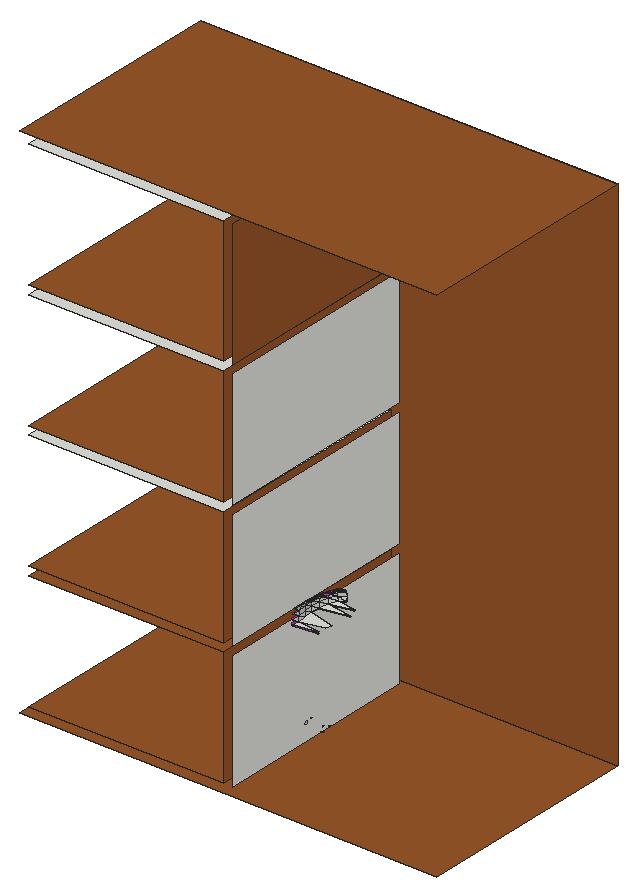
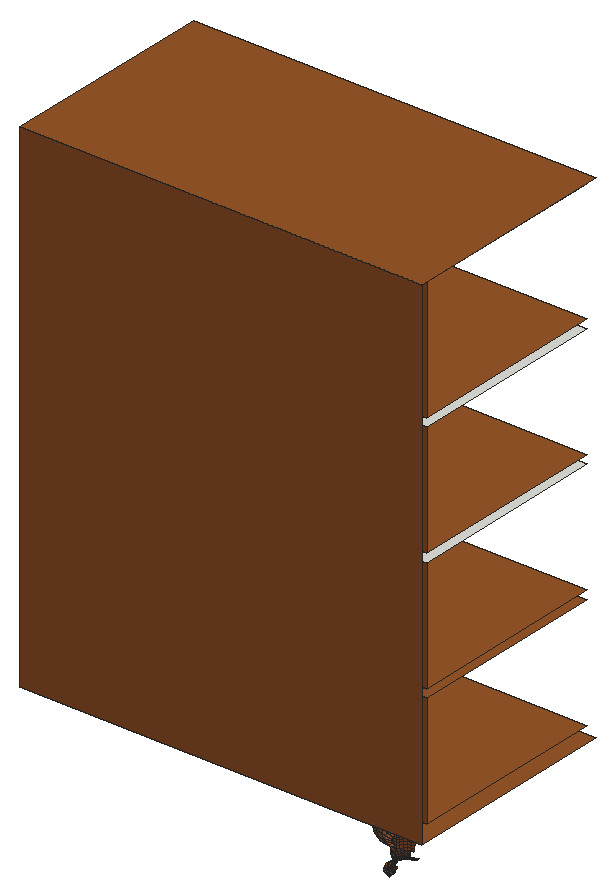
# SketchUp Ruby script. Lengths in inches.
U = 1.inch
M = Sketchup.active_model
def pt(a) = Geom::Point3d.new(a.map { |v| v * U })
def face(e, loops, mat)
  f = e.add_face(loops[0].map { |a| pt(a) })
  loops[1..].each { |l| e.add_face(l.map { |a| pt(a) }).erase! }
  f.material = f.back_material = mat if mat
  f
end
# faces: each face lists its corners as indices into pts; further lists are holes
def faces(e, pts, list, mat = nil) = list.each { |f| face(e, (f[0].is_a?(Array) ? f : [f]).map { |l| l.map { |i| pts[i] } }, mat) }
# xy, xz, yz: faces in a plane at the given z, y or x. An outline is a flat list of corners, or four numbers for a rectangle; further outlines are holes
def ring(l) = l.size == 4 ? [[l[0], l[1]], [l[2], l[1]], [l[2], l[3]], [l[0], l[3]]] : l.each_slice(2).to_a
def flat(e, list, mat, &to3) = list.each { |f| face(e, (f[0].is_a?(Array) ? f : [f]).map { |l| ring(l).map { |u, v| to3.(u, v) } }, mat) }
def xy(e, z, list, mat = nil) = flat(e, list, mat) { |x, y| [x, y, z] }
def xz(e, y, list, mat = nil) = flat(e, list, mat) { |x, z| [x, y, z] }
def yz(e, x, list, mat = nil) = flat(e, list, mat) { |y, z| [x, y, z] }
def lines(e, pts, list) = list.each { |a, b| e.add_line(pt(pts[a]), pt(pts[b])) }
# prism: a flat outline (further loops are holes) pulled along v
def prism(e, loops, v, mat = nil)
  f = face(e, loops, mat); d = Geom::Vector3d.new(v.map { |x| x * U })
  f.pushpull(f.normal.samedirection?(d) ? d.length : -d.length)
end
def box(e, o, s, mat = nil) = prism(e, [[o, [o[0] + s[0], o[1], o[2]], [o[0] + s[0], o[1] + s[1], o[2]], [o[0], o[1] + s[1], o[2]]]], [0, 0, s[2]], mat)
def at(x, y, z, deg = 0) = Geom::Transformation.translation(pt([x, y, z])) * Geom::Transformation.rotation(ORIGIN, Z_AXIS, deg.degrees)
def axes(o, x, y, z) = Geom::Transformation.new([*x, 0, *y, 0, *z, 0, *pt(o).to_a, 1])
def part(name) = M.definitions.add(name)
# library, detail: a bought-in or finely detailed component or shape, given as its bounding box
def library(name, o, s) = part(name).tap { |d| box(d.entities, o, s) }
def detail(e, o, s) = box(e.add_group.entities, o, s)
def put(e, d, t, mat = nil) = e.add_instance(d, t).tap { |i| i.material = mat if mat }
def group(e, t, mat = nil) = e.add_group.tap { |g| g.transformation = t; g.material = mat if mat }.entities
root = M.entities
M.materials.add("[Color K04]").color = [255, 50, 255]
M.materials.add("[Wood Cherry Original]").color = [152, 86, 42]
xy(root,13.078,[[154.901,46.115,202.901,72.115]],"[Wood Cherry Original]")
xy(root,14.078,[[155.901,46.115,178.354,70.115]],"[Wood Cherry Original]")
xy(root,27.578,[[155.901,46.115,178.354,70.115]],"[Wood Cherry Original]")
xy(root,28.578,[[155.901,46.115,178.354,70.115]],"[Wood Cherry Original]")
xy(root,42.078,[[155.901,46.115,178.354,70.115]])
xy(root,43.078,[[155.901,46.115,178.354,70.115]],"[Wood Cherry Original]")
xy(root,56.578,[[155.901,46.115,178.354,70.115]])
xy(root,57.578,[[155.901,46.115,178.354,70.115]],"[Wood Cherry Original]")
xy(root,72.078,[[155.901,46.115,178.354,70.115]])
xy(root,73.078,[[154.901,46.115,202.901,72.115]],"[Wood Cherry Original]")
xz(root,70.115,[[155.901,14.078,178.354,27.578],[155.901,28.578,178.354,42.078],[155.901,43.078,178.354,56.578],[155.901,57.578,178.354,72.078]],"[Wood Cherry Original]")
xz(root,72.115,[[154.901,13.078,202.901,73.078]],"[Wood Cherry Original]")
yz(root,178.354,[[46.115,14.078,70.115,27.578],[46.115,28.578,70.115,42.078],[46.115,43.078,70.115,56.578],[46.115,57.578,70.115,72.078]],"[Wood Cherry Original]")
yz(root,179.354,[[46.115,14.078,70.115,27.578],[46.115,28.578,70.115,42.078],[46.115,43.078,70.115,56.578]])
yz(root,179.354,[[46.115,57.578,70.115,72.078]],"[Wood Cherry Original]")
p = [[161.28,64.741,6.002],[161.299,64.59,6],[161.839,64.733,6],[161.782,64.873,6.002],[161.261,64.888,6.029],[161.725,65.011,6.029],
  [162.324,65.01,6],[162.232,65.131,6.002],[161.243,65.029,6.082],[161.671,65.142,6.082],[162.142,65.249,6.029],[162.056,65.362,6.082],
  [162.72,65.403,6],[162.6,65.496,6.002],[162.482,65.587,6.029],[162.37,65.674,6.082],[163.001,65.886,6],[162.861,65.944,6.002],
  [162.724,66.002,6.029],[162.593,66.057,6.082],[162.998,66.445,6.002],[162.85,66.465,6.029],[163.148,66.425,6],[162.709,66.484,6.082],
  [163,66.964,6.002],[162.852,66.945,6.029],[163.15,66.983,6],[162.711,66.927,6.082],[162.729,67.409,6.029],[162.598,67.355,6.082],
  [162.867,67.466,6.002],[163.007,67.523,6],[162.491,67.826,6.029],[162.378,67.74,6.082],[162.61,67.916,6.002],[162.73,68.008,6],
  [162.153,68.166,6.029],[162.066,68.054,6.082],[162.244,68.284,6.002],[162.337,68.404,6],[161.738,68.408,6.029],[161.683,68.277,6.082],
  [161.796,68.545,6.002],[161.275,68.534,6.029],[161.256,68.393,6.082],[161.854,68.685,6],[161.295,68.682,6.002],[161.315,68.832,6],
  [161.226,65.159,6.158],[161.622,65.263,6.158],[161.977,65.466,6.158],[162.267,65.754,6.158],[162.473,66.107,6.158],[162.58,66.502,6.158],
  [162.582,66.911,6.158],[162.477,67.306,6.158],[162.274,67.661,6.158],[161.986,67.951,6.158],[161.633,68.157,6.158],[161.238,68.264,6.158],
  [161.212,65.273,6.255],[161.578,65.37,6.255],[161.907,65.558,6.255],[162.176,65.825,6.255],[162.366,66.152,6.255],[162.466,66.517,6.255],
  [162.467,66.896,6.255],[162.371,67.262,6.255],[162.182,67.591,6.255],[161.916,67.86,6.255],[161.588,68.05,6.255],[161.223,68.15,6.255],
  [161.2,65.369,6.37],[161.541,65.459,6.37],[161.848,65.635,6.37],[162.099,65.884,6.37],[162.277,66.189,6.37],[162.37,66.53,6.37],
  [162.371,66.884,6.37],[162.281,67.225,6.37],[162.105,67.532,6.37],[161.856,67.783,6.37],[161.551,67.961,6.37],[161.21,68.054,6.37],
  [161.19,65.444,6.501],[161.513,65.529,6.501],[161.803,65.694,6.501],[162.04,65.93,6.501],[162.208,66.218,6.501],[162.295,66.54,6.501],
  [162.297,66.874,6.501],[162.212,67.197,6.501],[162.046,67.487,6.501],[161.811,67.724,6.501],[161.522,67.892,6.501],[161.2,67.979,6.501],
  [161.493,65.576,6.642],[161.772,65.735,6.642],[161.999,65.961,6.642],[162.16,66.238,6.642],[162.245,66.547,6.642],[162.246,66.868,6.642],
  [162.164,67.178,6.642],[162.005,67.456,6.642],[161.779,67.683,6.642],[161.502,67.844,6.642],[161.193,67.929,6.642],[161.484,65.6,6.79],
  [161.756,65.756,6.79],[161.979,65.977,6.79],[162.137,66.248,6.79],[162.219,66.551,6.79],[162.22,66.864,6.79],[162.14,67.168,6.79],
  [161.984,67.44,6.79],[161.763,67.663,6.79],[161.492,67.821,6.79],[161.484,65.6,6.94],[161.756,65.756,6.94],[161.979,65.977,6.94],
  [162.137,66.248,6.94],[162.219,66.551,6.94],[162.22,66.864,6.94],[162.14,67.168,6.94],[161.985,67.44,6.94],[161.763,67.663,6.94],
  [161.492,67.821,6.94],[161.494,65.575,7.088],[161.772,65.735,7.088],[162,65.961,7.088],[162.161,66.238,7.088],[162.245,66.547,7.088],
  [162.247,66.868,7.088],[162.165,67.178,7.088],[162.006,67.456,7.088],[161.78,67.684,7.088],[161.503,67.845,7.088],[161.513,65.527,7.229],
  [161.804,65.693,7.229],[162.041,65.929,7.229],[162.209,66.218,7.229],[162.297,66.54,7.229],[162.298,66.874,7.229],[162.213,67.197,7.229],
  [162.047,67.488,7.229],[161.811,67.725,7.229],[161.523,67.893,7.229],[161.193,67.929,7.088],[161.2,67.981,7.229],[161.204,65.332,7.509],
  [161.19,65.442,7.229],[161.556,65.425,7.509],[161.871,65.605,7.509],[162.129,65.861,7.509],[162.312,66.175,7.509],[162.407,66.525,7.509],
  [162.408,66.888,7.509],[162.316,67.24,7.509],[162.135,67.555,7.509],[161.879,67.813,7.509],[161.566,67.996,7.509],[161.215,68.091,7.509],
  [161.214,65.256,7.801],[161.584,65.354,7.801],[161.917,65.544,7.801],[162.189,65.814,7.801],[162.382,66.145,7.801],[162.482,66.515,7.801],
  [162.484,66.898,7.801],[162.386,67.268,7.801],[162.196,67.601,7.801],[161.926,67.873,7.801],[161.595,68.066,7.801],[161.225,68.166,7.801],
  [161.219,65.217,8.099],[161.599,65.317,8.099],[161.941,65.513,8.099],[162.22,65.79,8.099],[162.418,66.13,8.099],[162.522,66.51,8.099],
  [162.523,66.903,8.099],[162.423,67.284,8.099],[162.227,67.625,8.099],[161.95,67.904,8.099],[161.61,68.102,8.099],[161.231,68.206,8.099],
  [161.219,65.214,8.4],[161.601,65.315,8.4],[161.943,65.511,8.4],[162.223,65.788,8.4],[162.421,66.129,8.4],[162.524,66.509,8.4],
  [162.526,66.903,8.4],[162.425,67.285,8.4],[162.23,67.627,8.4],[161.952,67.907,8.4],[161.611,68.105,8.4],[161.231,68.209,8.4],
  [161.215,65.248,8.699],[161.588,65.346,8.699],[161.922,65.538,8.699],[162.196,65.809,8.699],[162.39,66.142,8.699],[162.491,66.514,8.699],
  [162.492,66.899,8.699],[162.394,67.272,8.699],[162.203,67.606,8.699],[161.931,67.88,8.699],[161.598,68.074,8.699],[161.226,68.175,8.699],
  [161.206,65.318,8.992],[161.561,65.411,8.992],[161.879,65.594,8.992],[162.14,65.852,8.992],[162.325,66.169,8.992],[162.421,66.523,8.992],
  [162.422,66.89,8.992],[162.329,67.245,8.992],[162.146,67.563,8.992],[161.888,67.824,8.992],[161.571,68.009,8.992],[161.217,68.105,8.992],
  [161.295,64.621,9.209],[161.827,64.762,9.209],[162.305,65.035,9.209],[162.695,65.422,9.209],[162.972,65.898,9.209],[163.117,66.429,9.209],
  [163.119,66.979,9.209],[162.979,67.511,9.209],[162.705,67.989,9.209],[162.318,68.379,9.209],[161.842,68.656,9.209],[161.311,68.801,9.209],
  [161.368,64.047,9.659],[162.047,64.226,9.659],[162.655,64.574,9.659],[163.153,65.068,9.659],[163.506,65.674,9.659],[163.691,66.351,9.659],
  [163.693,67.053,9.659],[163.514,67.731,9.659],[163.166,68.34,9.659],[162.672,68.837,9.659],[162.066,69.19,9.659],[161.389,69.375,9.659],
  [162.213,52.916,10.284],[162.066,52.565,9.659],[161.389,52.75,9.659],[161.44,53.127,10.284],[161.417,63.67,10.284],[162.191,63.874,10.284],
  [162.886,64.271,10.284],[163.454,64.835,10.284],[163.857,65.527,10.284],[164.068,66.3,10.284],[164.071,67.101,10.284],[163.866,67.875,10.284],
  [163.469,68.57,10.284],[162.905,69.138,10.284],[162.213,69.541,10.284],[161.44,69.752,10.284],[162.986,52.618,11.001],[162.905,52.513,10.284],
  [162.264,53.039,11.001],[161.458,53.258,11.001],[161.433,63.538,11.001],[162.241,63.751,11.001],[162.966,64.166,11.001],[163.559,64.754,11.001],
  [163.98,65.476,11.001],[164.199,66.282,11.001],[164.202,67.118,11.001],[163.989,67.925,11.001],[163.574,68.65,11.001],[162.986,69.243,11.001],
  [162.264,69.664,11.001],[161.458,69.883,11.001],[162.905,52.513,11.719],[162.213,52.916,11.719],[161.44,53.127,11.719],[161.417,63.67,11.719],
  [162.191,63.874,11.719],[162.886,64.271,11.719],[163.454,64.835,11.719],[163.857,65.527,11.719],[164.068,66.3,11.719],[164.071,67.101,11.719],
  [163.866,67.875,11.719],[163.469,68.57,11.719],[162.905,69.138,11.719],[162.213,69.541,11.719],[161.44,69.752,11.719],[162.066,52.565,12.343],
  [161.389,52.75,12.343],[161.368,64.047,12.343],[162.047,64.226,12.343],[162.655,64.574,12.343],[163.153,65.068,12.343],[163.506,65.674,12.343],
  [163.691,66.351,12.343],[163.693,67.053,12.343],[163.514,67.731,12.343],[163.166,68.34,12.343],[162.672,68.837,12.343],[162.066,69.19,12.343],
  [161.389,69.375,12.343],[161.295,64.621,12.793],[161.827,64.762,12.793],[162.305,65.035,12.793],[162.695,65.422,12.793],[162.972,65.898,12.793],
  [163.117,66.429,12.793],[163.119,66.979,12.793],[162.979,67.511,12.793],[162.705,67.989,12.793],[162.318,68.379,12.793],[161.842,68.656,12.793],
  [161.311,68.801,12.793],[161.028,66.712,12.668],[161.559,66.301,12.967],[161.647,66.453,12.967],[161.693,66.622,12.967],[161.694,66.797,12.967],
  [161.649,66.967,12.967],[161.562,67.119,12.967],[161.206,65.318,13.01],[161.561,65.411,13.01],[161.879,65.594,13.01],[162.14,65.852,13.01],
  [162.325,66.169,13.01],[162.421,66.523,13.01],[162.422,66.89,13.01],[162.329,67.245,13.01],[162.146,67.563,13.01],[161.888,67.824,13.01],
  [161.571,68.009,13.01],[161.217,68.105,13.01],[161.283,66.091,12.967],[161.435,66.178,12.967],[161.439,67.243,12.967],[161.287,67.331,12.967],
  [182.188,55.649,16.547],[182.227,55.647,16.536],[182.23,55.619,16.551],[182.238,55.192,16.782],[182.265,55.191,16.776],[182.267,55.159,16.791],
  [182.622,55.951,17.203],[182.622,55.951,17.202],[182.578,56.229,16.991],[182.626,55.95,17.209],[182.465,55.217,17.364],[182.463,55.267,17.336],
  [182.469,55.292,17.358],[182.461,55.291,17.323],[182.469,55.303,17.357],[182.133,53.346,18.609],[182.175,53.074,18.475],[182.176,53.069,18.4375],
  [182.121,53.433,18.333],[182.181,53.929,18.688],[182.165,53.931,18.688],[182.17,53.968,18.692],[182.19,53.986,18.693],[184.101,52.64,28.66],
  [181.454,52.216,28.66],[181.341,53.115,28.578],[181.375,52.203,28.74],[181.262,53.099,28.658],[181.165,54.137,28.578],[181.085,54.13,28.658],
  [180.983,55.197,28.658],[181.063,55.195,28.578],[181.135,56.291,28.578],[181.055,56.299,28.658],[181.268,57.367,28.698],[181.349,57.354,28.616],
  [184.381,56.88,28.579],[181.691,58.217,28.762],[181.793,58.205,28.679],[184.005,57.948,28.62],[181.262,53.099,28.873],[181.375,52.203,28.956],
  [181.392,53.129,28.709],[181.507,52.228,28.791],[184.048,52.64,28.791],[181.37,53.113,29.332],[181.485,52.206,29.372],[181.085,54.13,28.873],
  [184.019,53.67,28.71],[184.183,54.437,28.709],[181.12,55.196,28.708],[181.22,54.145,28.708],[181.219,54.153,29.33],[180.983,55.197,28.873],
  [181.105,55.215,29.333],[181.055,56.299,28.873],[181.191,56.281,28.708],[181.177,56.306,29.332],[181.268,57.367,28.913],[181.403,57.329,28.745],
  [184.326,56.863,28.708],[181.385,57.356,29.331],[181.835,58.149,28.802],[183.958,57.902,28.745],[181.691,58.217,28.978],[182.459,58.695,28.813],
  [182.48,58.615,28.722],[181.782,58.164,29.329],[182.495,58.543,28.843],[182.459,58.695,29.029],[182.489,58.607,29.328],[181.345,52.1875,29.381],
  [181.23,53.093,29.338],[181.079,54.135,29.338],[180.964,55.212,29.338],[181.037,56.325,29.338],[181.251,57.403,29.338],[181.679,58.261,29.338],
  [182.454,58.744,29.338],[181.449,52.234,29.968],[181.298,53.11,29.893],[181.436,53.13,29.865],[181.586,52.254,29.937],[181.147,54.123,29.855],
  [181.284,54.14,29.822],[181.02,55.168,29.855],[181.15,55.167,29.8],[181.091,56.249,29.855],[181.218,56.233,29.795],[181.33,57.36,29.855],
  [181.419,57.257,29.791],[181.809,58.048,29.79],[181.714,58.131,29.855],[182.5,58.481,29.785],[182.468,58.6,29.855],[181.582,53.153,30.356],
  [181.449,54.14,30.273],[181.509,55.104,30.165],[181.485,56.168,30.081],[181.676,57.176,30.036],[182.006,57.871,30.058],[182.567,58.217,30.042],
  [181.597,52.301,30.554],[181.465,53.139,30.457],[181.717,52.316,30.457],[181.341,54.131,30.389],[181.459,55.11,30.315],[181.415,56.181,30.204],
  [181.653,57.288,30.178],[181.948,57.919,30.179],[182.549,58.292,30.161],[182.161,56.634,30.173],[182.241,57.075,30.139],[182.506,57.831,30.159],
  [181.757,55.773,30.181],[182.243,56.261,30.209],[181.413,54.136,30.356],[181.512,55.102,30.255],[181.765,55.734,30.333],[181.782,55.725,30.255],
  [182.246,56.207,30.357],[182.253,56.2,30.277],[182.149,56.645,30.352],[182.245,57.259,30.327],[182.381,57.864,30.282],[181.541,53.148,30.433],
  [181.673,52.313,30.532]]
faces(root,p,[[0,1,2,3],[4,0,3,5],[3,2,6,7],[8,4,5,9],[5,3,7,10],[9,5,10,11],[7,6,12,13],[10,7,13,14],
  [11,10,14,15],[13,12,16,17],[14,13,17,18],[15,14,18,19],[18,17,20,21],[17,16,22,20],[19,18,21,23],[21,20,24,25],
  [20,22,26,24],[23,21,25,27],[27,25,28,29],[25,24,30,28],[24,26,31,30],[29,28,32,33],[28,30,34,32],[30,31,35,34],
  [33,32,36,37],[32,34,38,36],[34,35,39,38],[37,36,40,41],[36,38,42,40],[41,40,43,44],[38,39,45,42],[40,42,46,43],
  [42,45,47,46],[48,8,9,49],[49,9,11,50],[50,11,15,51],[51,15,19,52],[52,19,23,53],[53,23,27,54],[54,27,29,55],
  [55,29,33,56],[56,33,37,57],[57,37,41,58],[58,41,44,59],[60,48,49,61],[61,49,50,62],[62,50,51,63],[63,51,52,64],
  [64,52,53,65],[65,53,54,66],[66,54,55,67],[67,55,56,68],[68,56,57,69],[69,57,58,70],[70,58,59,71],[72,60,61,73],
  [73,61,62,74],[74,62,63,75],[75,63,64,76],[76,64,65,77],[77,65,66,78],[78,66,67,79],[79,67,68,80],[80,68,69,81],
  [81,69,70,82],[82,70,71,83],[84,72,73,85],[85,73,74,86],[86,74,75,87],[87,75,76,88],[88,76,77,89],[89,77,78,90],
  [90,78,79,91],[91,79,80,92],[92,80,81,93],[93,81,82,94],[94,82,83,95],[96,85,86,97],[97,86,87,98],[98,87,88,99],
  [99,88,89,100],[100,89,90,101],[101,90,91,102],[102,91,92,103],[103,92,93,104],[104,93,94,105],[105,94,95,106],[107,96,97,108],
  [108,97,98,109],[109,98,99,110],[110,99,100,111],[111,100,101,112],[112,101,102,113],[113,102,103,114],[114,103,104,115],[115,104,105,116],
  [117,107,108,118],[118,108,109,119],[119,109,110,120],[120,110,111,121],[121,111,112,122],[122,112,113,123],[123,113,114,124],[124,114,115,125],
  [125,115,116,126],[127,117,118,128],[128,118,119,129],[129,119,120,130],[130,120,121,131],[131,121,122,132],[132,122,123,133],[133,123,124,134],
  [134,124,125,135],[135,125,126,136],[137,127,128,138],[138,128,129,139],[139,129,130,140],[140,130,131,141],[141,131,132,142],[142,132,133,143],
  [143,133,134,144],[144,134,135,145],[145,135,136,146],[146,136,147,148],[149,150,137,151],[151,137,138,152],[152,138,139,153],[153,139,140,154],
  [154,140,141,155],[155,141,142,156],[156,142,143,157],[157,143,144,158],[158,144,145,159],[159,145,146,160],[160,146,148,161],[162,149,151,163],
  [163,151,152,164],[164,152,153,165],[165,153,154,166],[166,154,155,167],[167,155,156,168],[168,156,157,169],[169,157,158,170],[170,158,159,171],
  [171,159,160,172],[172,160,161,173],[174,162,163,175],[175,163,164,176],[176,164,165,177],[177,165,166,178],[178,166,167,179],[179,167,168,180],
  [180,168,169,181],[181,169,170,182],[182,170,171,183],[183,171,172,184],[184,172,173,185],[186,174,175,187],[187,175,176,188],[188,176,177,189],
  [189,177,178,190],[190,178,179,191],[191,179,180,192],[192,180,181,193],[193,181,182,194],[194,182,183,195],[195,183,184,196],[196,184,185,197],
  [198,186,187,199],[199,187,188,200],[200,188,189,201],[201,189,190,202],[202,190,191,203],[203,191,192,204],[204,192,193,205],[205,193,194,206],
  [206,194,195,207],[207,195,196,208],[208,196,197,209],[210,198,199,211],[211,199,200,212],[212,200,201,213],[213,201,202,214],[214,202,203,215],
  [215,203,204,216],[216,204,205,217],[217,205,206,218],[218,206,207,219],[219,207,208,220],[220,208,209,221],[222,210,211,223],[223,211,212,224],
  [224,212,213,225],[225,213,214,226],[226,214,215,227],[227,215,216,228],[228,216,217,229],[229,217,218,230],[230,218,219,231],[231,219,220,232],
  [232,220,221,233],[234,222,223,235],[235,223,224,236],[236,224,225,237],[237,225,226,238],[238,226,227,239],[239,227,228,240],[240,228,229,241],
  [241,229,230,242],[242,230,231,243],[243,231,232,244],[244,232,233,245],[246,247,248,249],[250,234,235,251],[251,235,236,252],[252,236,237,253],
  [253,237,238,254],[254,238,239,255],[255,239,240,256],[256,240,241,257],[257,241,242,258],[258,242,243,259],[259,243,244,260],[260,244,245,261],
  [262,263,246,264],[264,246,249,265],[266,250,251,267],[267,251,252,268],[268,252,253,269],[269,253,254,270],[270,254,255,271],[271,255,256,272],
  [272,256,257,273],[273,257,258,274],[274,258,259,275],[275,259,260,276],[276,260,261,277],[278,262,264,279],[279,264,265,280],[281,266,267,282],
  [282,267,268,283],[283,268,269,284],[284,269,270,285],[285,270,271,286],[286,271,272,287],[287,272,273,288],[288,273,274,289],[289,274,275,290],
  [290,275,276,291],[291,276,277,292],[293,279,280,294],[295,281,282,296],[296,282,283,297],[297,283,284,298],[298,284,285,299],[299,285,286,300],
  [300,286,287,301],[301,287,288,302],[302,288,289,303],[303,289,290,304],[304,290,291,305],[305,291,292,306],[307,295,296,308],[308,296,297,309],
  [309,297,298,310],[310,298,299,311],[311,299,300,312],[312,300,301,313],[313,301,302,314],[314,302,303,315],[315,303,304,316],[316,304,305,317],
  [317,305,306,318],[319,320,321],[319,321,322],[319,322,323],[319,323,324],[319,324,325],[326,307,308,327],[327,308,309,328],
  [328,309,310,329],[329,310,311,330],[330,311,312,331],[331,312,313,332],[332,313,314,333],[333,314,315,334],[334,315,316,335],[335,316,317,336],
  [336,317,318,337],[338,327,328,339],[339,328,329,320],[320,329,330,321],[321,330,331,322],[322,331,332,323],[323,332,333,324],[324,333,334,325],
  [325,334,335,340],[340,335,336,341]],"[Wood Cherry Original]")
faces(root,p,[[342,343,344],[345,346,347],[348,349,350,351],[352,353,354],[355,356,354,353],[356,354,353,355],[357,358,359,360],[361,362,363,364],
  [384,385,386],[384,387,388],[390,391,392,393,384],[387,384,393],[393,394,387],[394,393,392],[392,396,394],[396,392,398],
  [398,399,396],[399,398,401],[402,401,398],[401,403,399],[403,401,404],[405,404,401],[404,409,403],[409,404,410],
  [410,412,409],[387,423,424],[426,423,387,394],[426,394,396],[396,428,426],[428,396,399],[399,430,428],[430,399,403],
  [403,432,430],[432,403,409],[409,433,432],[435,433,409,412],[437,423,426],[426,438,437],[438,426,428],[428,439,438],
  [439,428,430],[430,440,439],[440,430,432],[432,441,440],[441,432,433],[433,442,441],[442,433,435],[435,443,442],
  [423,437,446],[453,440,441],[441,454,453],[454,441,442],[455,442,443],[456,439,440],[457,456,440],[440,453,457],
  [442,455,454],[458,438,439],[439,459,458],[459,439,456],[456,461,459],[461,456,457],[457,463,461],[467,437,438],
  [438,458,467],[448,447,458],[458,459,448],[460,448,459],[459,461,460],[462,460,461],[461,463,462],[468,467,445],
  [437,467,468],[468,446,437],[447,445,467],[467,458,447]])
faces(root,p,[[365,366,367],[367,366,368,369],[370,367,369,371],[370,371,372],[372,373,370],[374,373,372,375],[374,375,376],[374,377,378],
  [376,377,374],[377,376,379],[377,380,381],[379,380,377],[382,369,368,383],[389,371,369,382],[395,372,371,389],[397,375,372,395],
  [400,376,375,397],[406,379,376,400],[380,379,407],[407,408,380],[411,407,379,406],[413,414,382],[389,382,414],[414,415,389],
  [395,389,415],[415,416,395],[417,397,395,416],[400,397,417],[417,418,400],[406,400,418],[418,419,406],[411,406,419],
  [419,420,411],[421,422,414],[415,414,422],[422,425,415],[416,415,425],[425,427,416],[429,417,416,427],[418,417,429],
  [429,431,418],[434,419,418,431],[436,420,419,434],[444,445,422],[425,422,445],[445,447,425],[427,425,447],[447,448,427],
  [429,427,448],[448,449,429],[431,429,449],[449,450,431],[434,431,450],[450,451,434],[436,434,451],[451,452,436],
  [449,448,460],[449,460,462],[462,464,449],[450,449,464],[464,465,450],[451,450,465],[465,466,451],[452,451,466]],"[Color K04]")
